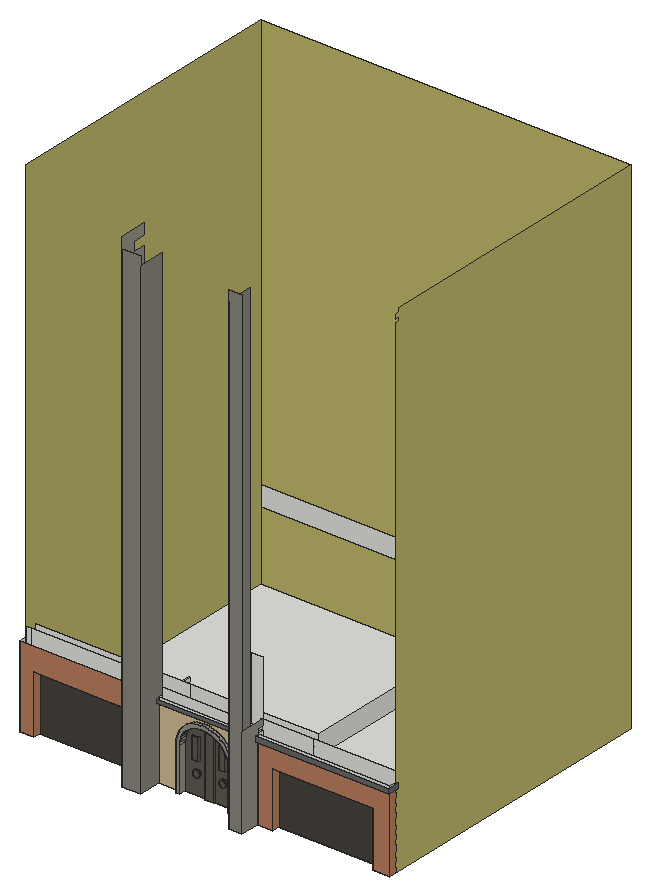
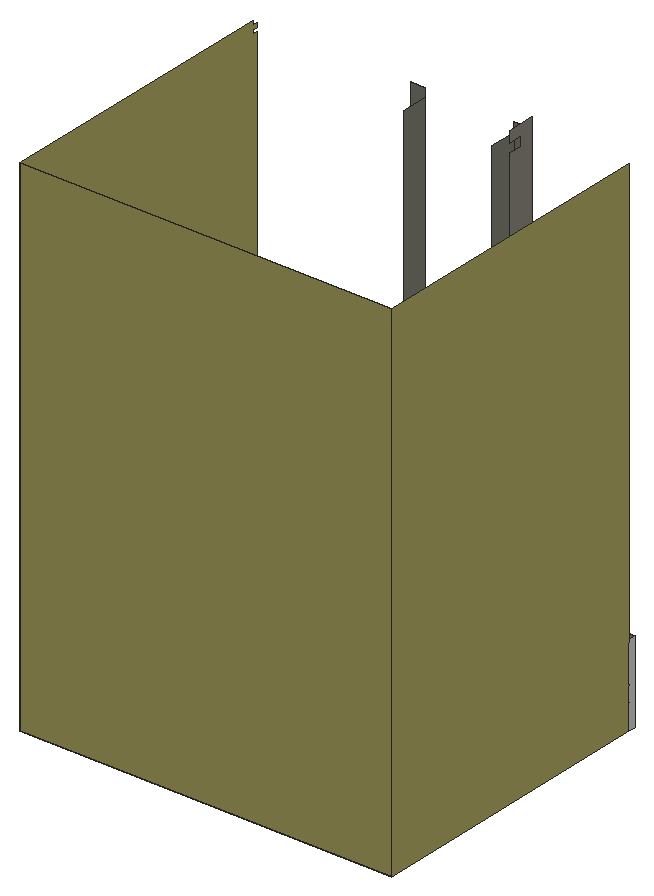
# SketchUp Ruby script. Lengths in inches.
U = 1.inch
M = Sketchup.active_model
def pt(a) = Geom::Point3d.new(a.map { |v| v * U })
def face(e, loops, mat)
  f = e.add_face(loops[0].map { |a| pt(a) })
  loops[1..].each { |l| e.add_face(l.map { |a| pt(a) }).erase! }
  f.material = f.back_material = mat if mat
  f
end
# faces: each face lists its corners as indices into pts; further lists are holes
def faces(e, pts, list, mat = nil) = list.each { |f| face(e, (f[0].is_a?(Array) ? f : [f]).map { |l| l.map { |i| pts[i] } }, mat) }
# xy, xz, yz: faces in a plane at the given z, y or x. An outline is a flat list of corners, or four numbers for a rectangle; further outlines are holes
def ring(l) = l.size == 4 ? [[l[0], l[1]], [l[2], l[1]], [l[2], l[3]], [l[0], l[3]]] : l.each_slice(2).to_a
def flat(e, list, mat, &to3) = list.each { |f| face(e, (f[0].is_a?(Array) ? f : [f]).map { |l| ring(l).map { |u, v| to3.(u, v) } }, mat) }
def xy(e, z, list, mat = nil) = flat(e, list, mat) { |x, y| [x, y, z] }
def xz(e, y, list, mat = nil) = flat(e, list, mat) { |x, z| [x, y, z] }
def yz(e, x, list, mat = nil) = flat(e, list, mat) { |y, z| [x, y, z] }
def lines(e, pts, list) = list.each { |a, b| e.add_line(pt(pts[a]), pt(pts[b])) }
# prism: a flat outline (further loops are holes) pulled along v
def prism(e, loops, v, mat = nil)
  f = face(e, loops, mat); d = Geom::Vector3d.new(v.map { |x| x * U })
  f.pushpull(f.normal.samedirection?(d) ? d.length : -d.length)
end
def box(e, o, s, mat = nil) = prism(e, [[o, [o[0] + s[0], o[1], o[2]], [o[0] + s[0], o[1] + s[1], o[2]], [o[0], o[1] + s[1], o[2]]]], [0, 0, s[2]], mat)
def at(x, y, z, deg = 0) = Geom::Transformation.translation(pt([x, y, z])) * Geom::Transformation.rotation(ORIGIN, Z_AXIS, deg.degrees)
def axes(o, x, y, z) = Geom::Transformation.new([*x, 0, *y, 0, *z, 0, *pt(o).to_a, 1])
def part(name) = M.definitions.add(name)
# library, detail: a bought-in or finely detailed component or shape, given as its bounding box
def library(name, o, s) = part(name).tap { |d| box(d.entities, o, s) }
def detail(e, o, s) = box(e.add_group.entities, o, s)
def put(e, d, t, mat = nil) = e.add_instance(d, t).tap { |i| i.material = mat if mat }
def group(e, t, mat = nil) = e.add_group.tap { |g| g.transformation = t; g.material = mat if mat }.entities
root = M.entities
M.materials.add("[0057_DarkKhaki]").color = [189, 183, 107]
M.materials.add("[0134_DimGray]").color = [105, 105, 105]
M.materials.add("[Cinder Block]").color = [186, 127, 95]
M.materials.add("[Cladding Weathered]").color = [71, 67, 61]
M.materials.add("[Cladding Weathered]1").color = [94, 89, 81]
M.materials.add("[Formica Beige]").color = [211, 187, 149]
M.materials.add("[Formica Graystone]").color = [137, 134, 124]
M.materials.add("[Formica Graystone]1").color = [149, 146, 135]
xy(root,0,[[370.55,6,370.74,43.6875],[259.78,37.6875,259.78,43.6875,226.6,43.6875,226.6,49.6875,4.9375,49.6875,4.9375,529.6875,608.5,529.6875,608.5,49.6875,370.74,49.6875,370.74,43.6875,349.65,43.6875,349.65,37.6875,343.65,37.6875,343.65,48.9375,314.85,48.9375,314.85,46.9375,300.03,46.9375,300.03,48.9375,265.78,48.9375,265.78,37.6875]])
xy(root,0,[[4.9375,37.6875,28.51,49.6875],[171.81,37.6875,197.35,49.6875],[392.7,37.6875,418.24,49.6875],[580.53,37.6875,608.5,49.6875]],"[Cinder Block]")
xy(root,0,[[197.35,6,197.35,49.6875,226.6,49.6875,226.6,43.6875,227.04,43.6875,227.04,6],[370.74,6,392.7,49.6875]],"[Formica Graystone]1")
xy(root,52.39,[[278.86,45.9375,289.3,48.9375],[322.86,45.9375,333.3,48.9375]])
xy(root,86.64,[[278.86,45.9375,289.3,48.9375],[322.86,45.9375,333.3,48.9375]],"[Cladding Weathered]1")
xy(root,90.21,[[418.24,37.6875,580.53,49.6875]],"[Cinder Block]")
xy(root,94.6,[[28.51,37.6875,171.81,49.6875]],"[Cinder Block]")
xy(root,106.3125,[[300.03,46.9375,302.75,49.6875],[300.03,49.6875,302.75,58.6875]])
xy(root,112.3125,[[299.83,37.6875,302.87,43.6875]],"[Formica Graystone]1")
xy(root,120,[[224.47,37.6875,224.47,49.6875,226.6,49.6875,226.6,43.6875,227.04,43.6875,227.04,37.6875],[370.55,37.6875,370.74,43.6875],[370.74,37.6875,374.55,49.6875],[226.6,43.6875,370.74,49.6875],[13.9375,49.6875,224.47,58.6875],
  [224.47,49.6875,226.6,58.6875],[226.6,49.6875,475.9375,58.6875],[224.47,58.6875,226.6,107.5]])
xy(root,120,[[227.04,37.6875,370.55,43.6875]],"[0134_DimGray]")
xy(root,124.15,[[389.32,31.6875,389.32,49.6875,392.7,49.6875,392.7,37.6875,608.5,37.6875,608.5,49.6875,611.75,49.6875,611.75,31.6875]],"[0134_DimGray]")
xz(root,6,[[197.35,0,227.04,787.6875],[370.55,0,392.7,787.6875]],"[Formica Graystone]")
xz(root,31.6875,[[389.32,124.15,611.75,131.98]],"[0134_DimGray]")
xz(root,37.6875,[[224.47,120,226.6,125.87],[226.6,120,227.04,125.87],[370.55,120,370.74,125.87],[370.74,120,374.55,125.87],[392.7,124.15,608.5,131.98]])
xz(root,37.6875,[[227.04,120,370.55,125.87]],"[0134_DimGray]")
xz(root,37.6875,[[4.9375,0,28.51,0,28.51,94.6,171.81,94.6,171.81,0,197.35,0,197.35,132.82,4.9375,132.82],[392.7,0,418.24,0,418.24,90.21,580.53,90.21,580.53,0,608.5,0,608.5,124.15,392.7,124.15]],"[Cinder Block]")
xz(root,37.6875,[[259.78,0,265.78,0,265.78,72.0625,266.07,76.53,266.94,80.93,268.38,85.17,270.36,89.1875,272.85,92.91,275.81,96.28,279.18,99.23,282.9,101.72,286.92,103.71,291.16,105.15,295.56,106.02,299.5,106.3125,300.625,106.4,302.75,106.3125,305.7,106.2,310.73,105.42,315.63,104.09,320.35,102.2,324.83,99.79,329,96.9,332.82,93.54,336.24,89.78,339.21,85.65,341.6875,81.22,343.65,76.53,343.65,0,349.65,0,349.65,77.74,347.09,83.85,344.28,88.88,340.91,93.5625,337.04,97.83,332.7,101.63,327.97,104.92,322.89,107.65,317.54,109.78,311.98,111.3,306.28,112.18,302.87,112.3125,299.83,112.3125,294.77,111.98,289.61,110.95,284.62,109.26,279.9,106.93,275.52,104,271.56,100.53,268.08,96.57,265.16,92.19,262.83,87.47,261.14,82.48,260.11,77.32,259.78,72.26]],"[Formica Graystone]1")
xz(root,43.6875,[[226.6,0,227.04,120],[370.55,0,370.74,120],[226.6,120,370.74,125.87]])
xz(root,43.6875,[[227.04,0,259.78,0,259.78,72.26,260.11,77.32,261.14,82.48,262.83,87.47,265.16,92.19,268.08,96.57,271.56,100.53,275.52,104,279.9,106.93,284.62,109.26,289.61,110.95,294.77,111.98,299.83,112.3125,302.87,112.3125,306.28,112.18,311.98,111.3,317.54,109.78,322.89,107.65,327.97,104.92,332.7,101.63,337.04,97.83,340.91,93.5625,344.28,88.88,347.09,83.85,349.65,77.74,349.65,0,370.55,0,370.55,120,227.04,120]],"[Formica Beige]")
xz(root,45.9375,[[285.99,27.4,287.43,27.59,288.77,28.14,289.92,29.03,290.81,30.18,291.36,31.52,291.55,32.96,291.36,34.4,290.81,35.74,289.92,36.89,288.77,37.78,287.43,38.33,285.99,38.52,284.55,38.33,283.21,37.78,282.06,36.89,281.17,35.74,280.62,34.4,280.43,32.96,280.62,31.52,281.17,30.18,282.06,29.03,283.21,28.14,284.55,27.59],[329.11,27.4,330.55,27.59,331.9,28.14,333.05,29.03,333.93,30.18,334.49,31.52,334.68,32.96,334.49,34.4,333.93,35.74,333.05,36.89,331.9,37.78,330.55,38.33,329.11,38.52,327.68,38.33,326.33,37.78,325.18,36.89,324.3,35.74,323.74,34.4,323.55,32.96,323.74,31.52,324.3,30.18,325.18,29.03,326.33,28.14,327.68,27.59],[278.86,52.39,289.3,86.64],[322.86,52.39,333.3,86.64]],"[Cladding Weathered]1")
xz(root,46.9375,[[300.03,0,314.85,0,314.85,104.3,310.73,105.42,305.7,106.2,302.75,106.3125,300.03,106.3125]],"[Cladding Weathered]1")
xz(root,48.9375,[[314.85,104.3,314.85,106.3125,302.75,106.3125,305.7,106.2,310.73,105.42]])
xz(root,48.9375,[[[265.78,0,300.03,0,300.03,106.3125,295.56,106.02,291.16,105.15,286.92,103.71,282.9,101.72,279.18,99.23,275.81,96.28,272.85,92.91,270.36,89.1875,268.38,85.17,266.94,80.93,266.07,76.53,265.78,72.0625],[278.86,52.39,289.3,86.64],[285.99,27.4,284.55,27.59,283.21,28.14,282.06,29.03,281.17,30.18,280.62,31.52,280.43,32.96,280.62,34.4,281.17,35.74,282.06,36.89,283.21,37.78,284.55,38.33,285.99,38.52,287.43,38.33,288.77,37.78,289.92,36.89,290.81,35.74,291.36,34.4,291.55,32.96,291.36,31.52,290.81,30.18,289.92,29.03,288.77,28.14,287.43,27.59]],[[314.85,0,343.65,0,343.65,76.53,341.6875,81.22,339.21,85.65,336.24,89.78,332.82,93.54,329,96.9,324.83,99.79,320.35,102.2,315.63,104.09,314.85,104.3],[322.86,52.39,333.3,86.64],[329.11,27.4,327.68,27.59,326.33,28.14,325.18,29.03,324.3,30.18,323.74,31.52,323.55,32.96,323.74,34.4,324.3,35.74,325.18,36.89,326.33,37.78,327.68,38.33,329.11,38.52,330.55,38.33,331.9,37.78,333.05,36.89,333.93,35.74,334.49,34.4,334.68,32.96,334.49,31.52,333.93,30.18,333.05,29.03,331.9,28.14,330.55,27.59]]],"[Cladding Weathered]1")
xz(root,49.6875,[[4.9375,0,4.9375,120,197.35,120,197.35,0,171.81,0,171.81,94.6,28.51,94.6,28.51,0],[370.74,0,392.7,120],[392.7,0,392.7,120,475.9375,120,475.9375,148.75,608.5,148.75,608.5,0,580.53,0,580.53,90.21,418.24,90.21,418.24,0],[295.56,106.02,300.03,106.3125,299.5,106.3125],[299.5,106.3125,302.75,106.3125,300.625,106.4],
  [4.9375,120,13.9375,148.75],[13.9375,120,197.35,148.75],[197.35,120,197.35,132.82,200.6,132.82,200.6,138.5625,197.35,138.5625,197.35,143.01,200.97,143.01,200.97,148.75,197.35,148.75,197.35,240,224.47,240,224.47,137.74,223.66,137.74,223.66,130.6875,224.47,130.6875,224.47,120],[224.47,120,226.6,125.87],[226.6,120,370.74,120,370.74,125.87,370.55,125.87,370.55,137.74,227.04,137.74,227.04,125.87,226.6,125.87],
  [374.55,120,374.55,130.6875,375.3,130.6875,375.3,137.74,374.55,137.74,374.55,240,392.7,240,392.7,148.75,387.45,148.75,387.45,139.38,392.7,139.38,392.7,131.98,389.32,131.98,389.32,124.15,392.7,124.15,392.7,120],[392.7,120,475.9375,148.75],[389.32,124.15,392.7,131.98],[608.5,124.15,611.75,131.98]])
xz(root,49.6875,[[28.51,0,171.81,94.6],[418.24,0,580.53,90.21]],"[Cladding Weathered]")
xz(root,49.6875,[[197.35,0,226.6,120]],"[Formica Graystone]1")
xz(root,58.6875,[[265.78,72.0625,265.78,120,343.65,120,343.65,76.53,341.6875,81.22,339.21,85.65,336.24,89.78,332.82,93.54,329,96.9,324.83,99.79,320.35,102.2,315.63,104.09,310.73,105.42,305.7,106.2,302.75,106.3125,300.03,106.3125,295.56,106.02,291.16,105.15,286.92,103.71,282.9,101.72,279.18,99.23,275.81,96.28,272.85,92.91,270.36,89.1875,268.38,85.17,266.94,80.93,266.07,76.53],[13.9375,120,265.78,151.875],[265.78,120,343.65,151.875],[343.65,120,475.9375,151.875]])
xz(root,107.5,[[224.47,120,226.6,125.87]])
xz(root,520.6875,[[13.9375,120,475.9375,151.875]])
xz(root,529.6875,[[4.9375,0,608.5,823.6875]],"[0057_DarkKhaki]")
yz(root,4.9375,[[37.6875,0,49.6875,132.82]])
yz(root,4.9375,[[49.6875,0,529.6875,823.6875]],"[0057_DarkKhaki]")
yz(root,28.51,[[37.6875,0,49.6875,94.6]],"[Cinder Block]")
yz(root,171.81,[[37.6875,0,49.6875,94.6]],"[Cinder Block]")
yz(root,197.35,[[37.6875,0,49.6875,120],[37.6875,120,49.6875,132.82]])
yz(root,197.35,[[6,0,6,805.29,49.6875,805.29,49.6875,787.6875,28.6875,787.6875,28.6875,772.09,49.6875,772.09,49.6875,143.01,37.6875,143.01,37.6875,0]],"[Formica Graystone]1")
yz(root,224.47,[[37.6875,120,49.6875,125.87],[49.6875,120,107.5,125.87]])
yz(root,226.6,[[43.6875,120,49.6875,125.87],[49.6875,120,107.5,125.87]])
yz(root,226.6,[[43.6875,0,49.6875,120]],"[Formica Graystone]1")
yz(root,227.04,[[6,0,43.6875,0,43.6875,120,37.6875,120,37.6875,125.87,49.6875,125.87,49.6875,772.09,6,772.09]],"[Formica Graystone]")
yz(root,259.78,[[37.6875,0,43.6875,72.26]],"[Formica Graystone]1")
yz(root,265.78,[[37.6875,0,48.9375,72.0625]],"[Formica Graystone]1")
yz(root,278.86,[[45.9375,52.39,48.9375,86.64]],"[Cladding Weathered]1")
yz(root,289.3,[[45.9375,52.39,48.9375,86.64]],"[Cladding Weathered]1")
yz(root,300.03,[[46.9375,0,48.9375,106.3125]],"[Cladding Weathered]1")
yz(root,314.85,[[46.9375,0,48.9375,104.3]],"[Cladding Weathered]1")
yz(root,322.86,[[45.9375,52.39,48.9375,86.64]],"[Cladding Weathered]1")
yz(root,333.3,[[45.9375,52.39,48.9375,86.64]],"[Cladding Weathered]1")
yz(root,343.65,[[37.6875,0,48.9375,76.53]],"[Formica Graystone]1")
yz(root,349.65,[[37.6875,0,43.6875,77.74]],"[Formica Graystone]1")
yz(root,370.55,[[6,0,6,772.09,49.6875,772.09,49.6875,125.87,37.6875,125.87,37.6875,120,43.6875,120,43.6875,0]],"[Formica Graystone]")
yz(root,370.74,[[43.6875,0,49.6875,120],[43.6875,120,49.6875,125.87]])
yz(root,374.55,[[37.6875,120,49.6875,125.87]])
yz(root,389.32,[[31.6875,124.15,49.6875,131.98]])
yz(root,392.7,[[37.6875,0,49.6875,120],[37.6875,120,49.6875,124.15],[37.6875,124.15,49.6875,131.98]])
yz(root,392.7,[[6,0,37.6875,0,37.6875,139.38,49.6875,139.38,49.6875,148.75,6,148.75]],"[Formica Graystone]1")
yz(root,418.24,[[37.6875,0,49.6875,90.21]],"[Cinder Block]")
yz(root,475.9375,[[58.6875,120,520.6875,151.875]])
yz(root,580.53,[[37.6875,0,49.6875,90.21]],"[Cinder Block]")
yz(root,608.5,[[37.6875,124.15,49.6875,131.98]])
yz(root,608.5,[[49.6875,0,529.6875,0,529.6875,823.6875,56.5625,823.6875,56.5625,816.49,49.6875,816.49,49.6875,809.61,56.5625,809.61,56.5625,804.58,49.6875,804.58]],"[0057_DarkKhaki]")
yz(root,608.5,[[37.6875,0,49.6875,124.15]],"[Cinder Block]")
yz(root,611.75,[[31.6875,124.15,49.6875,131.98]],"[0134_DimGray]")
p = [[284.55,48.9375,27.59],[285.99,48.9375,27.4],[285.99,45.9375,27.4],[284.55,45.9375,27.59],[287.43,48.9375,27.59],[287.43,45.9375,27.59],
  [327.68,48.9375,27.59],[329.11,48.9375,27.4],[329.11,45.9375,27.4],[327.68,45.9375,27.59],[330.55,48.9375,27.59],[330.55,45.9375,27.59],
  [283.21,48.9375,28.14],[283.21,45.9375,28.14],[288.77,48.9375,28.14],[288.77,45.9375,28.14],[326.33,48.9375,28.14],[326.33,45.9375,28.14],
  [331.9,48.9375,28.14],[331.9,45.9375,28.14],[282.06,48.9375,29.03],[282.06,45.9375,29.03],[289.92,48.9375,29.03],[289.92,45.9375,29.03],
  [325.18,48.9375,29.03],[325.18,45.9375,29.03],[333.05,48.9375,29.03],[333.05,45.9375,29.03],[281.17,48.9375,30.18],[281.17,45.9375,30.18],
  [290.81,48.9375,30.18],[290.81,45.9375,30.18],[324.3,48.9375,30.18],[324.3,45.9375,30.18],[333.93,48.9375,30.18],[333.93,45.9375,30.18],
  [280.62,48.9375,31.52],[280.62,45.9375,31.52],[291.36,48.9375,31.52],[291.36,45.9375,31.52],[323.74,48.9375,31.52],[323.74,45.9375,31.52],
  [334.49,48.9375,31.52],[334.49,45.9375,31.52],[280.43,48.9375,32.96],[280.43,45.9375,32.96],[291.55,48.9375,32.96],[291.55,45.9375,32.96],
  [323.55,48.9375,32.96],[323.55,45.9375,32.96],[334.68,48.9375,32.96],[334.68,45.9375,32.96],[280.62,48.9375,34.4],[280.62,45.9375,34.4],
  [291.36,48.9375,34.4],[291.36,45.9375,34.4],[323.74,48.9375,34.4],[323.74,45.9375,34.4],[334.49,48.9375,34.4],[334.49,45.9375,34.4],
  [281.17,48.9375,35.74],[281.17,45.9375,35.74],[290.81,48.9375,35.74],[290.81,45.9375,35.74],[324.3,48.9375,35.74],[324.3,45.9375,35.74],
  [333.93,48.9375,35.74],[333.93,45.9375,35.74],[282.06,48.9375,36.89],[282.06,45.9375,36.89],[289.92,48.9375,36.89],[289.92,45.9375,36.89],
  [325.18,48.9375,36.89],[325.18,45.9375,36.89],[333.05,48.9375,36.89],[333.05,45.9375,36.89],[283.21,48.9375,37.78],[283.21,45.9375,37.78],
  [288.77,48.9375,37.78],[288.77,45.9375,37.78],[326.33,48.9375,37.78],[326.33,45.9375,37.78],[331.9,48.9375,37.78],[331.9,45.9375,37.78],
  [284.55,48.9375,38.33],[284.55,45.9375,38.33],[287.43,48.9375,38.33],[287.43,45.9375,38.33],[327.68,48.9375,38.33],[327.68,45.9375,38.33],
  [330.55,48.9375,38.33],[330.55,45.9375,38.33],[285.99,48.9375,38.52],[285.99,45.9375,38.52],[329.11,48.9375,38.52],[329.11,45.9375,38.52],
  [266.07,48.9375,76.53],[266.07,37.6875,76.53],[265.78,37.6875,72.0625],[265.78,48.9375,72.0625],[265.78,58.6875,72.0625],[266.07,58.6875,76.53],
  [260.11,43.6875,77.32],[259.78,43.6875,72.26],[259.78,37.6875,72.26],[260.11,37.6875,77.32],[266.94,48.9375,80.93],[266.94,37.6875,80.93],
  [343.65,48.9375,76.53],[343.65,37.6875,76.53],[341.6875,37.6875,81.22],[341.6875,48.9375,81.22],[266.94,58.6875,80.93],[341.6875,58.6875,81.22],
  [343.65,58.6875,76.53],[261.14,43.6875,82.48],[261.14,37.6875,82.48],[349.65,43.6875,77.74],[347.09,43.6875,83.85],[347.09,37.6875,83.85],
  [349.65,37.6875,77.74],[268.38,48.9375,85.17],[268.38,37.6875,85.17],[268.38,58.6875,85.17],[339.21,37.6875,85.65],[339.21,48.9375,85.65],
  [339.21,58.6875,85.65],[262.83,43.6875,87.47],[262.83,37.6875,87.47],[344.28,43.6875,88.88],[344.28,37.6875,88.88],[270.36,48.9375,89.1875],
  [270.36,37.6875,89.1875],[270.36,58.6875,89.1875],[336.24,37.6875,89.78],[336.24,48.9375,89.78],[336.24,58.6875,89.78],[265.16,43.6875,92.19],
  [265.16,37.6875,92.19],[340.91,43.6875,93.5625],[340.91,37.6875,93.5625],[272.85,48.9375,92.91],[272.85,37.6875,92.91],[272.85,58.6875,92.91],
  [332.82,37.6875,93.54],[332.82,48.9375,93.54],[332.82,58.6875,93.54],[268.08,43.6875,96.57],[268.08,37.6875,96.57],[275.81,48.9375,96.28],
  [275.81,37.6875,96.28],[275.81,58.6875,96.28],[329,37.6875,96.9],[329,48.9375,96.9],[329,58.6875,96.9],[337.04,43.6875,97.83],
  [337.04,37.6875,97.83],[279.18,48.9375,99.23],[279.18,37.6875,99.23],[279.18,58.6875,99.23],[271.56,43.6875,100.53],[271.56,37.6875,100.53],
  [324.83,37.6875,99.79],[324.83,48.9375,99.79],[324.83,58.6875,99.79],[332.7,43.6875,101.63],[332.7,37.6875,101.63],[282.9,48.9375,101.72],
  [282.9,37.6875,101.72],[282.9,58.6875,101.72],[320.35,37.6875,102.2],[320.35,48.9375,102.2],[320.35,58.6875,102.2],[275.52,43.6875,104],
  [275.52,37.6875,104],[327.97,43.6875,104.92],[327.97,37.6875,104.92],[286.92,48.9375,103.71],[286.92,37.6875,103.71],[286.92,58.6875,103.71],
  [315.63,37.6875,104.09],[315.63,48.9375,104.09],[315.63,58.6875,104.09],[291.16,48.9375,105.15],[291.16,37.6875,105.15],[291.16,58.6875,105.15],
  [279.9,43.6875,106.93],[279.9,37.6875,106.93],[310.73,37.6875,105.42],[310.73,46.9375,105.42],[314.85,46.9375,104.3],[314.85,48.9375,104.3],
  [310.73,58.6875,105.42],[310.73,48.9375,105.42],[322.89,43.6875,107.65],[322.89,37.6875,107.65],[295.56,48.9375,106.02],[295.56,37.6875,106.02],
  [295.56,58.6875,106.02],[295.56,49.6875,106.02],[305.7,37.6875,106.2],[305.7,46.9375,106.2],[305.7,48.9375,106.2],[305.7,58.6875,106.2],
  [299.5,49.6875,106.3125],[300.625,49.6875,106.4],[300.625,37.6875,106.4],[299.5,37.6875,106.3125],[300.03,48.9375,106.3125],[300.03,49.6875,106.3125],
  [300.03,58.6875,106.3125],[302.75,49.6875,106.3125],[302.75,48.9375,106.3125],[302.75,46.9375,106.3125],[302.75,37.6875,106.3125],[302.75,58.6875,106.3125],
  [284.62,43.6875,109.26],[284.62,37.6875,109.26],[317.54,43.6875,109.78],[317.54,37.6875,109.78],[289.61,43.6875,110.95],[289.61,37.6875,110.95],
  [311.98,43.6875,111.3],[311.98,37.6875,111.3],[294.77,43.6875,111.98],[294.77,37.6875,111.98],[306.28,43.6875,112.18],[306.28,37.6875,112.18],
  [299.83,43.6875,112.3125],[299.83,37.6875,112.3125],[302.87,43.6875,112.3125],[302.87,37.6875,112.3125],[475.9375,58.6875,120],[484.9375,58.6875,120],
  [13.9375,520.6875,120],[13.9375,529.6875,120],[475.9375,520.6875,120],[475.9375,529.6875,120],[484.9375,520.6875,120],[4.9375,520.6875,120],
  [13.9375,58.6875,0],[13.9375,58.6875,120],[475.9375,58.6875,0],[475.9375,520.6875,0],[13.9375,520.6875,0]]
faces(root,p,[[0,1,2,3],[1,4,5,2],[6,7,8,9],[7,10,11,8],[12,0,3,13],[4,14,15,5],[16,6,9,17],[10,18,19,11],
  [20,12,13,21],[14,22,23,15],[24,16,17,25],[18,26,27,19],[28,20,21,29],[22,30,31,23],[32,24,25,33],[26,34,35,27],
  [36,28,29,37],[30,38,39,31],[40,32,33,41],[34,42,43,35],[44,36,37,45],[38,46,47,39],[48,40,41,49],[42,50,51,43],
  [52,44,45,53],[46,54,55,47],[56,48,49,57],[50,58,59,51],[60,52,53,61],[54,62,63,55],[64,56,57,65],[58,66,67,59],
  [68,60,61,69],[62,70,71,63],[72,64,65,73],[66,74,75,67],[76,68,69,77],[70,78,79,71],[80,72,73,81],[74,82,83,75],
  [84,76,77,85],[78,86,87,79],[88,80,81,89],[82,90,91,83],[92,84,85,93],[86,92,93,87],[94,88,89,95],[90,94,95,91]],"[Cladding Weathered]1")
faces(root,p,[[96,97,98,99],[102,103,104,105],[106,107,97,96],[108,109,110,111],[115,102,105,116],[117,118,119,120],[121,122,107,106],[111,110,124,125],
  [127,115,116,128],[118,129,130,119],[131,132,122,121],[125,124,134,135],[137,127,128,138],[129,139,140,130],[141,142,132,131],[135,134,144,145],
  [147,137,138,148],[149,150,142,141],[145,144,152,153],[139,155,156,140],[157,158,150,149],[160,147,148,161],[153,152,162,163],[155,165,166,156],
  [167,168,158,157],[163,162,170,171],[173,160,161,174],[165,175,176,166],[177,178,168,167],[171,170,180,181],[183,184,178,177],[186,173,174,187],
  [181,180,188,189,190,191],[175,194,195,176],[184,183,196,197],[189,188,200,201],[199,204,205,206,207,197,196],[205,211,212,213,201,200,214,206],[216,186,187,217],[194,218,219,195],
  [220,216,217,221],[218,222,223,219],[224,220,221,225],[222,226,227,223],[228,224,225,229],[226,230,231,227]],"[Formica Graystone]1")
faces(root,p,[[100,101,96,99],[101,112,106,96],[113,114,108,111],[112,123,121,106],[126,113,111,125],[123,133,131,121],[136,126,125,135],[133,143,141,131],
  [146,136,135,145],[143,151,149,141],[154,146,145,153],[151,159,157,149],[164,154,153,163],[159,169,167,157],[172,164,163,171],[169,179,177,167],
  [182,172,171,181],[179,185,183,177],[192,182,181,191,193],[193,191,190,189],[185,198,199,196,183],[202,193,189,201],[203,192,193,202],[208,209,199,196],
  [199,209,210,198],[212,202,201,213],[215,203,202,212,211]])
lines(root,p,[[232,233],[234,235],[236,237],[236,238],[234,239],[240,241],[242,232],[243,236],[244,234]])
